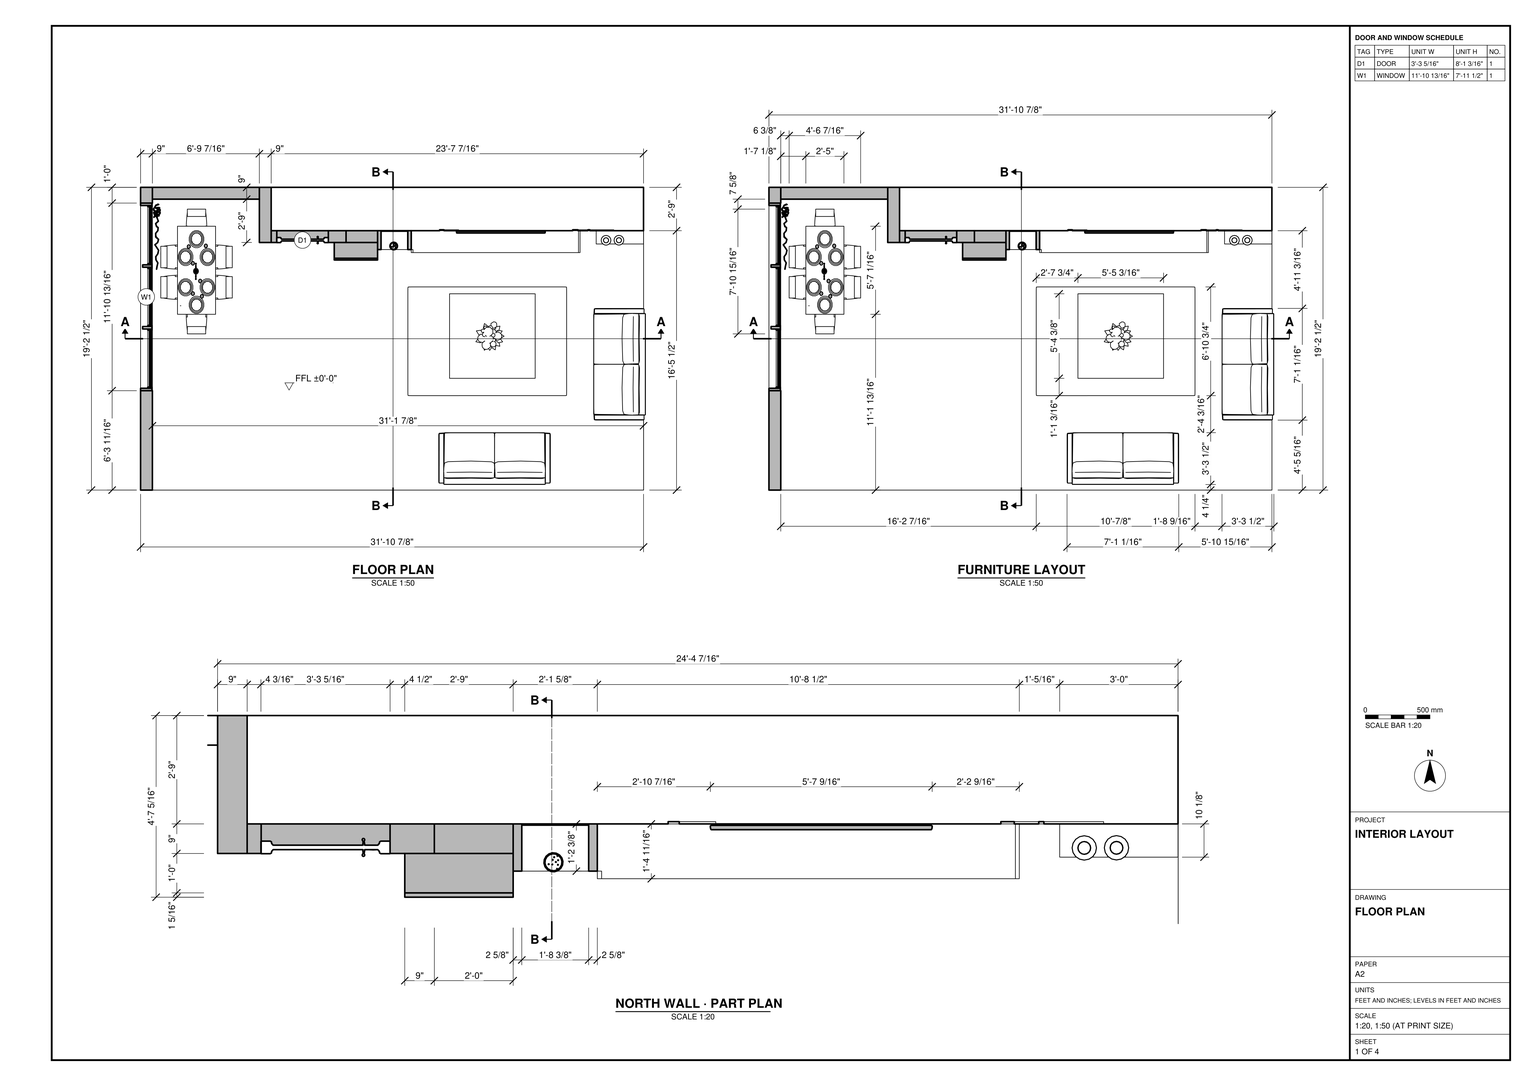
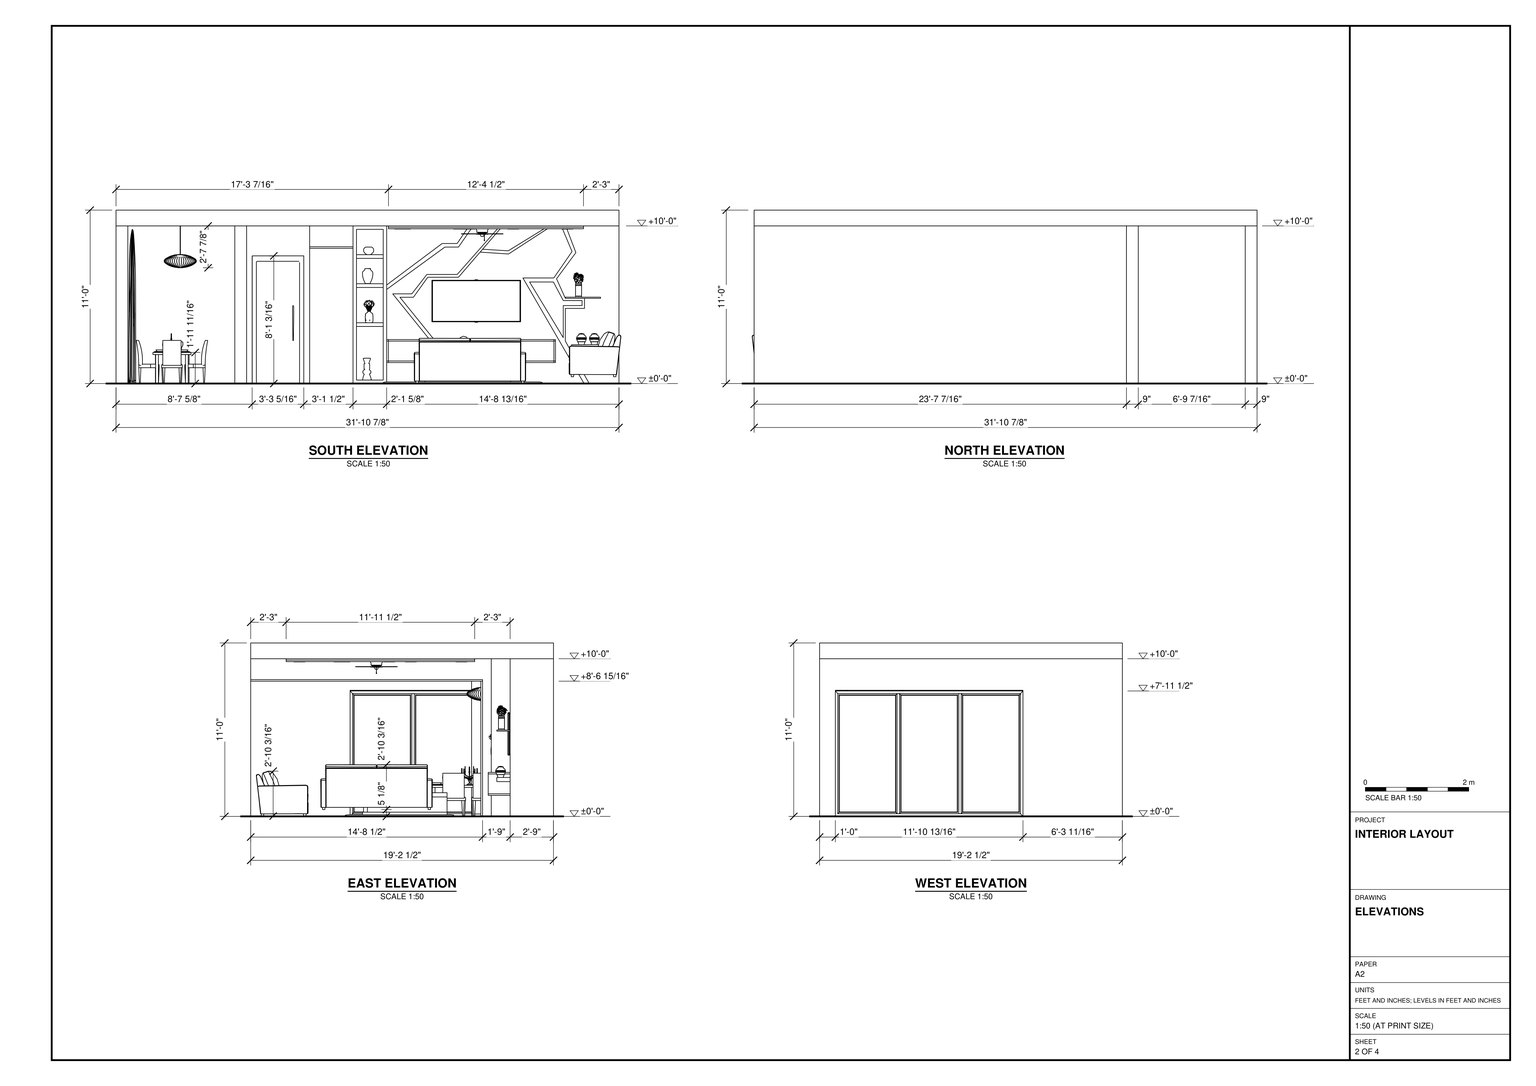
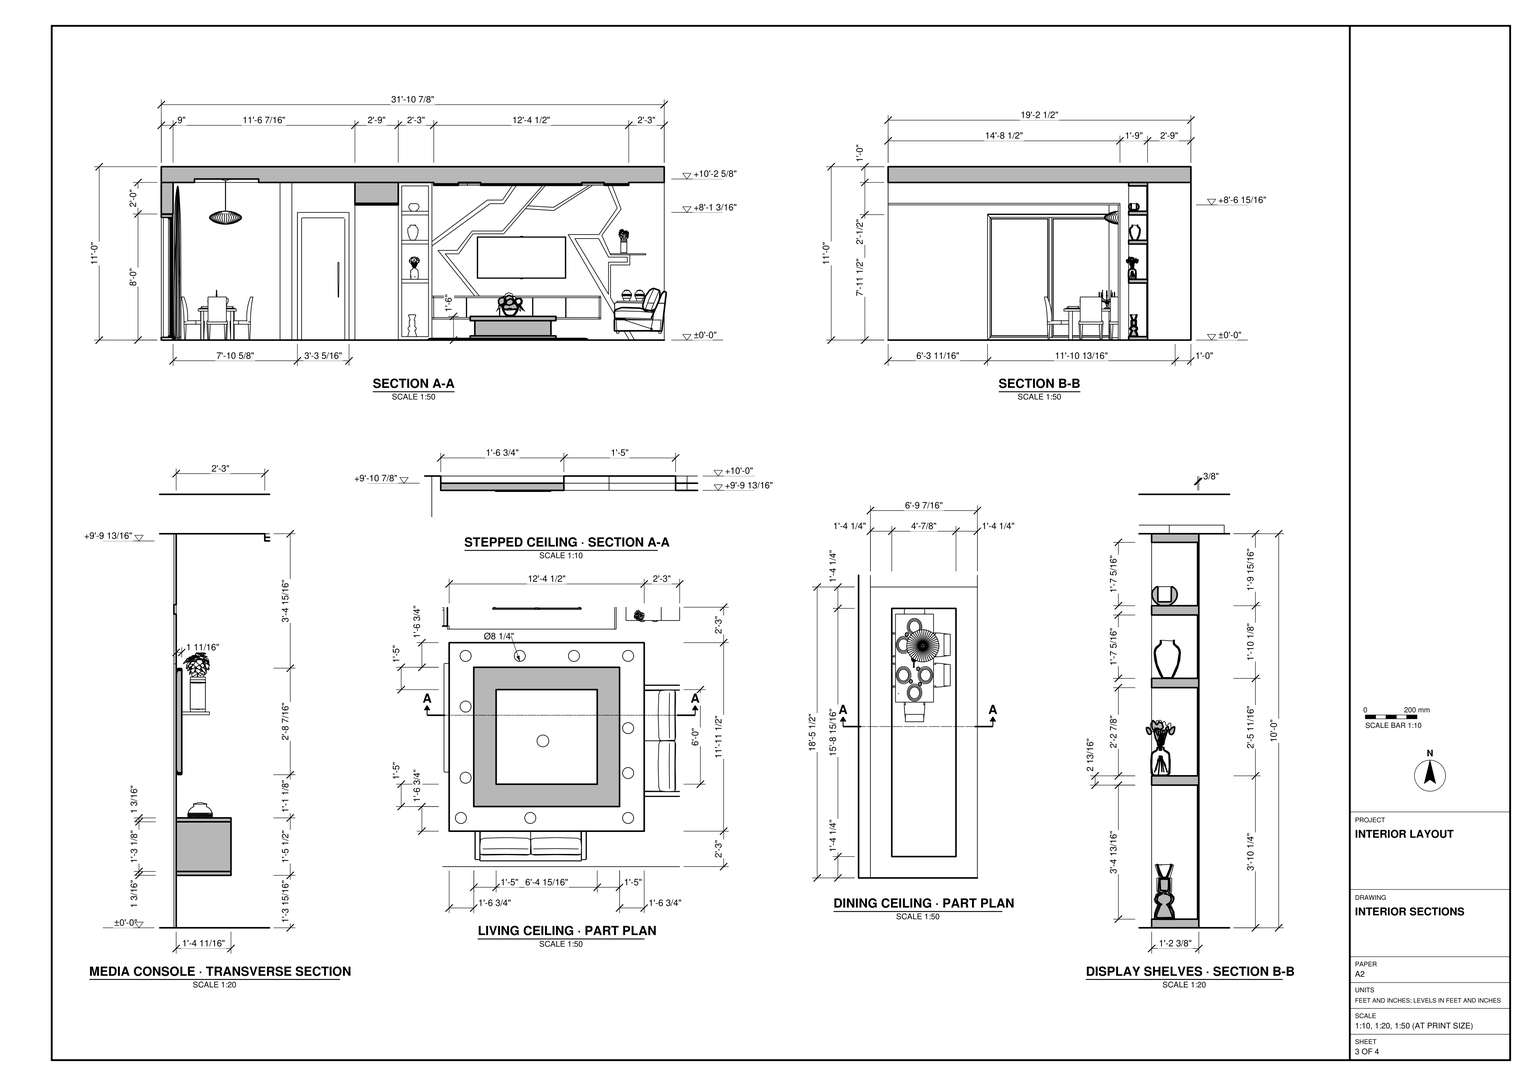
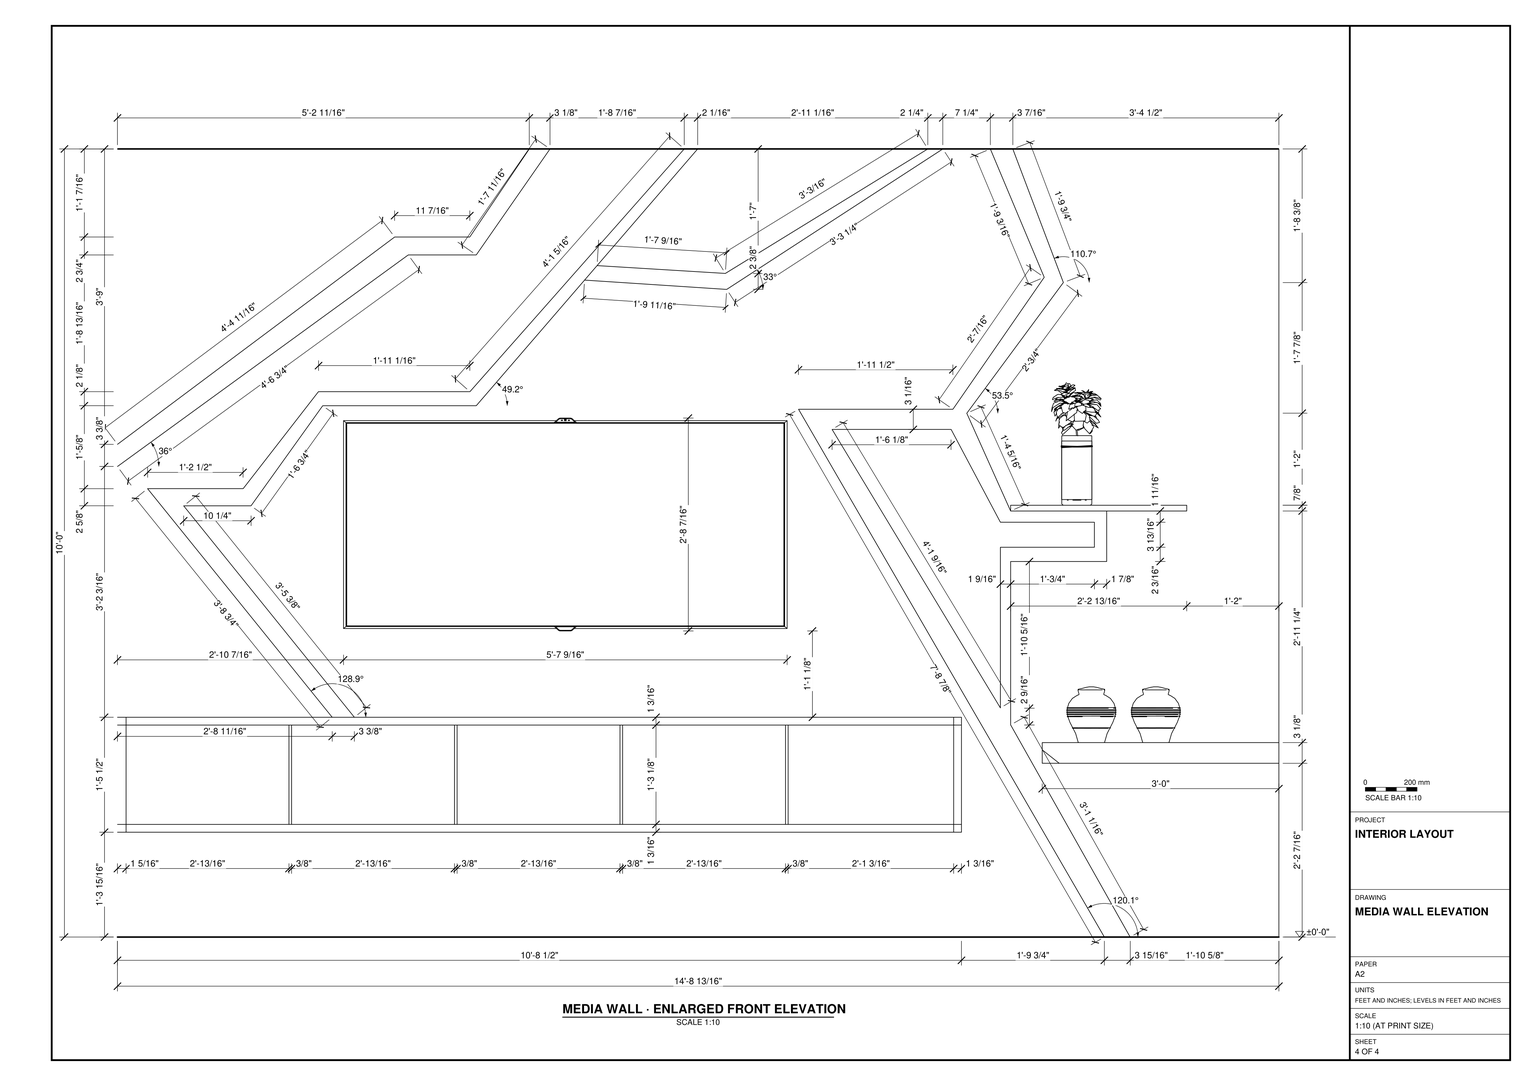
Build the furnished interior in SketchUp using task_files/diagram_01.pdf. Work in feet and inches. Set the finished floor at ±0'-0" and make the overall model 32'-3/8" along the x-axis, 19'-2 1/2" along the y-axis and 11'-0" high.

Follow the floor plan for the floor, the west window wall and the stepped north wall. Use the wall thicknesses shown, including the 9" wall returns. Fit the three-panel window beside the dining area and the single door in the north wall recess. Model the overhead slab with its main underside at +10'-0". Use the ceiling plans and sections to form the stepped rectangular ceiling over the living area and the long inset panel over the dining area.

Arrange the dining table and chairs by the window. Place the two sofas at right angles around the coffee table and rug. On the north wall, model the tall open display shelves, suspended media console, wall-mounted screen and angular wall detailing shown in elevation. Decor and loose items, including curtains, lights, the rug, tableware and shelf objects, may be any suitable library components.

Keep the walls, floor and overhead slab separate as groups or components. Make each furniture or joinery piece a separate group or component and use components for repeated parts. Save one SketchUp model as output_files/living_and_dining_interior_with_a_built_in_media_wall.skp.

# SketchUp Ruby script. Lengths in inches.
U = 1.inch
M = Sketchup.active_model
def pt(a) = Geom::Point3d.new(a.map { |v| v * U })
def face(e, loops, mat)
  f = e.add_face(loops[0].map { |a| pt(a) })
  loops[1..].each { |l| e.add_face(l.map { |a| pt(a) }).erase! }
  f.material = f.back_material = mat if mat
  f
end
# faces: each face lists its corners as indices into pts; further lists are holes
def faces(e, pts, list, mat = nil) = list.each { |f| face(e, (f[0].is_a?(Array) ? f : [f]).map { |l| l.map { |i| pts[i] } }, mat) }
# xy, xz, yz: faces in a plane at the given z, y or x. An outline is a flat list of corners, or four numbers for a rectangle; further outlines are holes
def ring(l) = l.size == 4 ? [[l[0], l[1]], [l[2], l[1]], [l[2], l[3]], [l[0], l[3]]] : l.each_slice(2).to_a
def flat(e, list, mat, &to3) = list.each { |f| face(e, (f[0].is_a?(Array) ? f : [f]).map { |l| ring(l).map { |u, v| to3.(u, v) } }, mat) }
def xy(e, z, list, mat = nil) = flat(e, list, mat) { |x, y| [x, y, z] }
def xz(e, y, list, mat = nil) = flat(e, list, mat) { |x, z| [x, y, z] }
def yz(e, x, list, mat = nil) = flat(e, list, mat) { |y, z| [x, y, z] }
def lines(e, pts, list) = list.each { |a, b| e.add_line(pt(pts[a]), pt(pts[b])) }
# prism: a flat outline (further loops are holes) pulled along v
def prism(e, loops, v, mat = nil)
  f = face(e, loops, mat); d = Geom::Vector3d.new(v.map { |x| x * U })
  f.pushpull(f.normal.samedirection?(d) ? d.length : -d.length)
end
def box(e, o, s, mat = nil) = prism(e, [[o, [o[0] + s[0], o[1], o[2]], [o[0] + s[0], o[1] + s[1], o[2]], [o[0], o[1] + s[1], o[2]]]], [0, 0, s[2]], mat)
def at(x, y, z, deg = 0) = Geom::Transformation.translation(pt([x, y, z])) * Geom::Transformation.rotation(ORIGIN, Z_AXIS, deg.degrees)
def axes(o, x, y, z) = Geom::Transformation.new([*x, 0, *y, 0, *z, 0, *pt(o).to_a, 1])
def part(name) = M.definitions.add(name)
# library, detail: a bought-in or finely detailed component or shape, given as its bounding box
def library(name, o, s) = part(name).tap { |d| box(d.entities, o, s) }
def detail(e, o, s) = box(e.add_group.entities, o, s)
def put(e, d, t, mat = nil) = e.add_instance(d, t).tap { |i| i.material = mat if mat }
def group(e, t, mat = nil) = e.add_group.tap { |g| g.transformation = t; g.material = mat if mat }.entities
root = M.entities
M.materials.add("Emissive").color = [230, 227, 173]
M.materials.add("[Color F02]").color = [204, 255, 153]
M.materials.add("[Sandstone]").color = [118, 81, 52]
M.materials.add("[Wood Veneer 01]").color = [120, 70, 37]
c1 = library("Dining Table",[54.55,57.53,0],[71.62,106.71,46.43])
c2 = library("Curtains 003",[-24.98,-2.79,0.01],[49.96,5.58,117.31])
c3 = library("Window 46-47",[-61.02,-2.17,0],[122.04,4.34,74.02])
c4 = library("Couch Potato Lite Sofa",[-42.52,-18.39,0],[85.04,39.49,34.18])
c5 = library("Pendant 001",[-12.3,-12.27,-34.51],[24.6,24.54,34.51])
c6 = library("Tlon Light 1950 Ceiling 152 010",[-38.39,-38.39,-3.78],[76.78,76.78,3.41])
c7 = library("Potted Basil 50-07",[-3.85,-3.53,0.03],[7.56,8,18.65])
c8 = library("Fan 90-20",[-15.86,-15.86,-9.19],[31.73,31.72,9.19])
c9 = library("Vase 014",[-3.77,-3.77,0],[7.54,7.54,8.49])
c10 = library("Rug 293 007",[-90.2,-61.78,-0.71],[180.4,123.56,1.82])
c11 = library("Door 243 053",[-21.6,-2.79,-0.07],[43.2,5.58,82.64])
c12 = library("Vase 296 007 003",[-3.87,-3.86,-0.02],[7.74,7.71,5.84])
c13 = library("Vase 293 004 008",[-3.27,-3.11,-0.05],[6.67,6.28,16.74])
c14 = library("Vase Tulips 12",[-3.9,-4.34,0],[7.8,8.68,17.22])
c15 = library("Vase 017",[-3.98,-3.95,0],[7.96,7.89,11.62])
c16 = library("Flat screen television",[0,1.41,1.14],[35.92,0.28,20.21])
c17 = library("Vase 008",[-10.64,-10.96,0.22],[21.74,21.78,17.78])
xy(root,0,[[0,0,9,75.6875],[9,0,382.92,0,382.92,197.5,360.23,197.5,360.23,198.1875,356.3,198.1875,356.3,197.5,206.05,197.5,206.05,183.125,180.42,183.125,180.42,175.1875,147.42,175.1875,147.42,188.5,142.94,188.5,142.94,197.5,103.69,197.5,103.69,188.5,90.42,188.5,90.42,221.5,9,221.5],[147.42,175.1875,156.42,176.5],[156.42,175.1875,180.42,176.5],[147.42,176.5,156.42,188.5],
  [156.42,176.5,180.42,188.5],[180.42,183.125,206.05,197.5],[90.42,188.5,99.42,230.5],[99.42,188.5,103.69,197.5],[142.94,188.5,156.42,197.5],
  [156.42,188.5,180.42,197.5],[99.42,197.5,356.3,197.5,356.3,198.1875,360.23,198.1875,360.23,197.5,382.875,197.5,382.875,230.5,99.42,230.5],[0,218.5,9,230.5],[9,221.5,90.42,230.5]])
xy(root,1.21,[[235.21,85.09,300.4,149.47]])
xy(root,2.63,[[183.06,183.125,203.42,197.125]],"[Wood Veneer 01]")
xy(root,3.21,[[235.21,85.09,238.71,149.47],[238.71,85.09,278.85,85.91],[278.85,85.09,278.85,88.84,297.9,88.84,297.9,87.59,300.4,87.59,300.4,85.09],[238.71,85.91,238.71,149.47,296.65,149.47,296.65,88.84,278.85,88.84,278.85,85.91],[297.9,87.59,297.9,88.84,296.65,88.84,296.65,149.47,300.4,149.47,300.4,87.59]])
xy(root,14.78,[[235.21,85.09,238.71,149.47],[238.71,85.09,278.85,85.91],[278.85,85.09,278.85,88.84,297.9,88.84,297.9,87.59,300.4,87.59,300.4,85.09],[238.71,85.91,238.71,149.47,296.65,149.47,296.65,88.84,278.85,88.84,278.85,85.91],[297.9,87.59,297.9,88.84,296.65,88.84,296.65,149.47,300.4,149.47,300.4,87.59]])
xy(root,15.96,[[206.05,180.8125,207.36,183.125],[207.36,180.8125,207.36,183.125,206.05,183.125,206.05,197.5,333.36,197.5,333.36,180.8125],[333.36,180.8125,334.55,197.5]],"[Wood Veneer 01]")
xy(root,17.15,[[206.05,180.8125,207.36,183.125],[207.36,180.8125,333.36,180.8125,333.36,197.5,206.05,197.5,206.05,183.125,207.36,183.125],[333.36,180.8125,334.55,197.5]])
xy(root,18.03,[[235.21,85.09,300.4,149.47]])
xy(root,26.46,[[346.85,187.375,349.4375,197.5],[349.4375,187.375,382.875,197.5]])
xy(root,29.61,[[346.85,187.375,382.875,197.5]])
xy(root,32.28,[[206.05,180.8125,207.36,183.125],[207.36,180.8125,207.36,183.125,206.05,183.125,206.05,197.5,333.36,197.5,333.36,180.8125],[333.36,180.8125,334.55,197.5]])
xy(root,33.46,[[238.74,197.5,242.12,198.1875]])
xy(root,33.46,[[206.05,180.8125,207.36,183.125],[207.36,180.8125,333.36,180.8125,333.36,197.5,206.05,197.5,206.05,183.125,207.36,183.125],[333.36,180.8125,334.55,197.5]],"[Wood Veneer 01]")
xy(root,43.44,[[183.06,195.125,203.42,197.125]],"Emissive")
xy(root,43.44,[[183.06,183.125,203.42,195.125]],"[Sandstone]")
xy(root,46.27,[[183.06,183.125,203.42,197.125]],"[Wood Veneer 01]")
xy(root,57.18,[[342.03,197.5,356.66,198.1875]],"Emissive")
xy(root,59.35,[[340.48,197.5,354.79,198.1875]],"Emissive")
xy(root,63.16,[[340.48,197.5,354.79,198.1875]],"Emissive")
xy(root,64.87,[[342.03,187.375,356.66,198.1875],[356.66,187.375,368.85,197.5]],"[Wood Veneer 01]")
xy(root,65.66,[[216.13,197.5,226.38,198.1875]],"Emissive")
xy(root,65.74,[[342.03,187.375,368.85,197.5]],"[Wood Veneer 01]")
xy(root,68.28,[[210.625,197.5,225.1875,198.1875]],"Emissive")
xy(root,73.13,[[183.06,195.125,203.42,197.125]],"Emissive")
xy(root,73.13,[[183.06,183.125,203.42,195.125]],"[Wood Veneer 01]")
xy(root,75.96,[[183.06,183.125,203.42,197.125]],"[Wood Veneer 01]")
xy(root,77.29,[[314.85,197.5,332.97,198.1875]],"Emissive")
xy(root,80.36,[[309.74,197.5,333.24,198.1875]],"Emissive")
xy(root,80.9,[[237.3,197.5,260.67,198.1875]],"Emissive")
xy(root,83.04,[[236.65,197.5,259.71,198.1875]],"Emissive")
xy(root,95.25,[[183.06,195.125,203.42,197.125]],"Emissive")
xy(root,95.25,[[183.06,183.125,203.42,195.125]],"[Wood Veneer 01]")
xy(root,96,[[0,75.6875,9,218.5]])
xy(root,97.1875,[[103.69,188.5,142.94,197.5]])
xy(root,98.08,[[183.06,183.125,203.42,197.125]],"[Wood Veneer 01]")
xy(root,102.92,[[147.42,175.1875,180.42,176.5]])
xy(root,102.92,[[147.42,0,180.42,175.1875]],"[Wood Veneer 01]")
xy(root,103.86,[[250.32,197.5,260.67,198.1875]],"Emissive")
xy(root,104.11,[[147.42,0,180.42,176.5]])
xy(root,106.59,[[248.25,197.5,259.69,198.1875]],"Emissive")
xy(root,117.37,[[183.06,195.125,203.42,197.125]],"Emissive")
xy(root,117.37,[[183.06,183.125,203.42,195.125]],"[Wood Veneer 01]")
xy(root,117.8125,[[[207.41,26.99,355.89,170.51],[226.16,45.74,337.14,151.76]],[243.17,62.74,320.13,134.76]])
xy(root,118.91,[[[207.41,26.99,355.89,170.51],[226.16,45.74,337.14,151.76]],[243.17,62.74,320.13,134.76]])
xy(root,120,[[0,0,9,230.5],[[9,0,90.42,221.5],[25.28,16.28,74.14,205.22]],[90.42,0,99.42,188.5],[99.42,0,147.42,188.5],[147.42,0,156.42,188.5],
  [156.42,0,180.42,188.5],[[180.42,0,180.42,183.125,206.05,183.125,206.05,197.5,268.75,197.5,268.75,198.1875,271.9,198.1875,271.9,197.5,292.34,197.5,292.34,198.1875,294.39,198.1875,294.39,197.5,329.43,197.5,329.43,198.1875,331.71,198.1875,331.71,197.5,338.94,197.5,338.94,198.1875,342.36,198.1875,342.36,197.5,382.875,197.5,382.875,0],[207.41,26.99,355.89,170.51]],[[226.16,45.74,337.14,151.76],[243.17,62.74,320.13,134.76]],[180.42,183.125,206.05,197.5],[90.42,188.5,99.42,230.5],
  [99.42,188.5,156.42,197.5],[156.42,188.5,180.42,197.5],[156.42,188.5,180.42,197.5],[99.42,197.5,99.42,230.5,382.875,230.5,382.875,197.5,342.36,197.5,342.36,198.1875,338.94,198.1875,338.94,197.5,331.71,197.5,331.71,198.1875,329.43,198.1875,329.43,197.5,294.39,197.5,294.39,198.1875,292.34,198.1875,292.34,197.5,271.9,197.5,271.9,198.1875,268.75,198.1875,268.75,197.5],[9,221.5,90.42,230.5]])
xy(root,122.625,[[25.28,16.28,74.14,205.22]])
xy(root,132,[[0,0,382.875,230.5]])
xz(root,0,[[0,0,9,120],[147.42,102.92,180.42,104.11],[147.42,104.11,180.42,120],[0,120,382.875,132]])
xz(root,16.28,[[25.28,120,74.14,122.625]])
xz(root,26.99,[[207.41,117.8125,355.89,118.91]])
xz(root,26.99,[[207.41,118.91,355.89,120]],"Emissive")
xz(root,45.74,[[226.16,117.8125,337.14,118.91],[226.16,118.91,337.14,120]])
xz(root,62.74,[[243.17,117.8125,320.13,118.91]])
xz(root,62.74,[[243.17,118.91,320.13,120]],"Emissive")
xz(root,75.6875,[[0,0,9,96]])
xz(root,85.09,[[235.21,1.21,300.4,3.21],[235.21,14.78,300.4,18.03]])
xz(root,85.91,[[238.71,3.21,278.85,14.78]])
xz(root,88.84,[[278.85,3.21,296.65,14.78]])
xz(root,134.76,[[243.17,117.8125,244.91,118.91],[244.91,117.8125,267.4,118.91],[267.4,117.8125,304.73,118.91],[304.73,117.8125,315.37,118.91],[315.37,117.8125,320.13,118.91]])
xz(root,134.76,[[243.17,118.91,244.91,120],[244.91,118.91,267.4,120],[267.4,118.91,304.73,120],[304.73,118.91,315.37,120],[315.37,118.91,320.13,120]],"Emissive")
xz(root,149.47,[[235.21,1.21,300.4,3.21],[238.71,3.21,296.65,14.78],[235.21,14.78,300.4,18.03]])
xz(root,151.76,[[226.16,117.8125,233.04,118.91],[233.04,117.8125,244.91,118.91],[244.91,117.8125,267.4,118.91],[267.4,117.8125,304.73,118.91],[304.73,117.8125,315.37,118.91],
  [315.37,117.8125,337.14,118.91]])
xz(root,151.76,[[226.16,118.91,233.04,120],[233.04,118.91,244.91,120],[244.91,118.91,267.4,120],[267.4,118.91,304.73,120],[304.73,118.91,315.37,120],
  [315.37,118.91,337.14,120]],"Emissive")
xz(root,170.51,[[207.41,117.8125,233.04,118.91],[233.04,117.8125,244.91,118.91],[244.91,117.8125,267.4,118.91],[267.4,117.8125,304.73,118.91],[304.73,117.8125,315.37,118.91],
  [315.37,117.8125,355.89,118.91]])
xz(root,170.51,[[207.41,118.91,233.04,120],[233.04,118.91,244.91,120],[244.91,118.91,267.4,120],[267.4,118.91,304.73,120],[304.73,118.91,315.37,120],
  [315.37,118.91,355.89,120]],"Emissive")
xz(root,175.1875,[[147.42,0,180.42,102.92]],"[Wood Veneer 01]")
xz(root,176.5,[[147.42,0,180.42,102.92],[147.42,102.92,180.42,104.11]])
xz(root,180.8125,[[207.36,17.15,232.16,32.28],[232.16,17.15,232.5625,32.28],[232.5625,17.15,257.36,32.28],[257.36,17.15,257.76,32.28],[257.76,17.15,282.5625,32.28],
  [282.5625,17.15,282.96,32.28],[282.96,17.15,307.76,32.28],[307.76,17.15,308.16,32.28],[308.16,17.15,333.36,32.28]])
xz(root,180.8125,[[206.05,15.96,207.36,17.15],[207.36,15.96,333.36,17.15],[333.36,15.96,334.55,17.15],[206.05,17.15,207.36,32.28],[333.36,17.15,334.55,32.28],
  [206.05,32.28,207.36,33.46],[207.36,32.28,333.36,33.46],[333.36,32.28,334.55,33.46]],"[Wood Veneer 01]")
xz(root,183.125,[[206.05,15.96,207.36,17.15],[206.05,17.15,207.36,32.28],[206.05,32.28,207.36,33.46]])
xz(root,183.125,[[[180.42,0,206.05,120],[183.06,2.63,203.42,117.37]],[183.06,43.44,203.42,46.27],[183.06,73.13,203.42,75.96],[183.06,95.25,203.42,98.08]],"[Wood Veneer 01]")
xz(root,187.375,[[346.85,26.46,349.4375,26.46,346.85,28.5],[349.4375,26.46,382.875,26.46,382.875,29.61,346.85,29.61,346.85,28.5]])
xz(root,187.375,[[342.03,64.87,368.85,65.74]],"[Wood Veneer 01]")
xz(root,188.5,[[90.42,0,99.42,120],[99.42,0,103.69,0,103.69,97.1875,142.94,97.1875,142.94,0,147.42,0,147.42,120,99.42,120],[147.42,0,156.42,120],[156.42,0,180.42,120]])
xz(root,197.125,[[183.06,2.63,203.42,43.44],[183.06,46.27,203.42,73.13],[183.06,75.96,203.42,95.25],[183.06,98.08,203.42,117.37]],"[Wood Veneer 01]")
xz(root,197.5,[[99.42,0,103.69,120],[103.69,0,142.94,97.1875],[142.94,0,156.42,120],[156.42,0,180.42,120],[180.42,0,206.05,120],
  [206.05,0,356.3,0,309.74,80.36,333.24,80.36,347.15,100.46,338.94,120,331.71,120,298.81,98.61,277.17,100.03,260.67,80.9,237.3,80.9,226.38,65.66,216.13,65.66,242.12,33.46,334.55,33.46,334.55,15.96,206.05,15.96],[382.875,0,382.92,0,382.875,0.04],[206.05,15.96,333.36,17.15],[333.36,15.96,334.55,17.15],[206.05,17.15,333.36,32.28],
  [333.36,17.15,334.55,32.28],[346.85,26.46,346.85,28.5,349.4375,26.46],[349.4375,26.46,346.85,28.5,346.85,29.61,382.875,29.61,382.875,26.46],[206.05,32.28,333.36,33.46],[333.36,32.28,334.55,33.46],
  [340.48,34.89,340.48,59.35,354.79,59.35,354.79,63.16,340.48,63.16,332.97,77.29,314.85,77.29],[206.05,75.02,248.25,106.59,259.69,106.59,268.75,120,206.05,120],[103.69,97.1875,142.94,120]])
xz(root,197.5,[[206.05,33.46,238.74,33.46,210.625,68.28,225.1875,68.28,236.65,83.04,259.71,83.04,292.34,120,271.9,120,260.67,103.86,250.32,103.86,206.05,71.65]],"[Color F02]")
xz(root,197.5,[[[360.23,0,382.875,0,382.875,0.04,382.92,0,382.875,0,382.875,26.46,346.85,26.46,346.85,29.61,382.875,29.61,382.875,120,342.36,120,350.0625,99.66,335.36,79.75,342.03,64.87,342.03,65.74,368.85,65.74,368.85,64.87,356.66,64.87,356.66,57.18,342.03,57.18,342.03,32.31],[346.85,26.46,346.85,28.5,349.4375,26.46]],[298.6,101.04,329.43,120,294.39,120,280.99,104.46,279.07,102.23]],"[Sandstone]")
xz(root,198.1875,[[[356.3,0,360.23,0,342.03,32.31,342.03,57.18,356.66,57.18,356.66,64.87,342.03,64.87,335.36,79.75,350.0625,99.66,342.36,120,338.94,120,347.15,100.46,333.24,80.36,309.74,80.36],[340.48,34.89,314.85,77.29,332.97,77.29,340.48,63.16,354.79,63.16,354.79,59.35,340.48,59.35]],[238.74,33.46,242.12,33.46,216.13,65.66,226.38,65.66,237.3,80.9,260.67,80.9,277.17,100.03,279.07,102.23,280.99,104.46,294.39,120,292.34,120,259.71,83.04,236.65,83.04,225.1875,68.28,210.625,68.28],[206.05,71.65,250.32,103.86,260.67,103.86,271.9,120,268.75,120,259.69,106.59,248.25,106.59,206.05,75.02],[298.81,98.61,331.71,120,329.43,120,298.6,101.04,279.07,102.23,277.17,100.03]])
xz(root,205.22,[[25.28,120,74.14,122.625]])
xz(root,218.5,[[0,0,9,96]])
xz(root,221.5,[[9,0,90.42,120]])
xz(root,230.5,[[0,0,9,120],[9,0,90.42,120],[90.42,0,99.42,120],[99.42,0,382.875,120],[0,120,382.875,132]])
yz(root,0,[[0,0,0,120,230.5,120,230.5,0,218.5,0,218.5,96,75.6875,96,75.6875,0],[0,120,230.5,132]])
yz(root,9,[[0,0,75.6875,0,75.6875,96,218.5,96,218.5,0,221.5,0,221.5,120,0,120],[221.5,0,230.5,120]])
yz(root,25.28,[[16.28,120,205.22,122.625]])
yz(root,74.14,[[16.28,120,188.5,122.625],[188.5,120,205.22,122.625]])
yz(root,90.42,[[188.5,0,221.5,120],[221.5,0,230.5,120]])
yz(root,99.42,[[188.5,0,197.5,120],[197.5,0,230.5,120]])
yz(root,103.69,[[188.5,0,197.5,97.1875]])
yz(root,142.94,[[188.5,0,197.5,97.1875]])
yz(root,147.42,[[176.5,0,176.5,104.11,0,104.11,0,120,188.5,120,188.5,0]])
yz(root,147.42,[[175.1875,0,176.5,102.92],[0,102.92,176.5,104.11]],"[Wood Veneer 01]")
yz(root,156.42,[[188.5,0,197.5,120]])
yz(root,180.42,[[176.5,0,183.125,0,183.125,120,0,120,0,104.11,176.5,104.11],[183.125,0,188.5,120],[188.5,0,197.5,120]])
yz(root,180.42,[[175.1875,0,176.5,102.92],[0,102.92,176.5,104.11]],"[Wood Veneer 01]")
yz(root,183.06,[[183.125,2.63,197.125,43.44],[183.125,46.27,197.125,73.13],[183.125,75.96,197.125,95.25],[183.125,98.08,197.125,117.37]],"[Wood Veneer 01]")
yz(root,203.42,[[183.125,2.63,197.125,15.96],[183.125,15.96,197.125,17.15],[183.125,17.15,197.125,32.28],[183.125,32.28,197.125,33.46],[183.125,33.46,197.125,43.44],
  [183.125,46.27,197.125,73.13],[183.125,75.96,197.125,95.25],[183.125,98.08,197.125,117.37]],"[Wood Veneer 01]")
yz(root,206.05,[[183.125,0,197.5,15.96],[183.125,15.96,197.5,17.15],[183.125,17.15,197.5,32.28],[183.125,32.28,197.5,33.46]])
yz(root,206.05,[[197.5,71.65,198.1875,75.02]],"Emissive")
yz(root,206.05,[[180.8125,15.96,183.125,17.15],[180.8125,17.15,183.125,32.28],[180.8125,32.28,183.125,33.46],[183.125,33.46,197.5,120]],"[Wood Veneer 01]")
yz(root,207.36,[[180.8125,15.96,183.125,17.15],[180.8125,17.15,183.125,32.28],[180.8125,32.28,183.125,33.46]])
yz(root,207.41,[[26.99,117.8125,170.51,118.91]])
yz(root,207.41,[[26.99,118.91,170.51,120]],"Emissive")
yz(root,226.16,[[45.74,117.8125,151.76,118.91]])
yz(root,226.16,[[45.74,118.91,151.76,120]],"Emissive")
yz(root,235.21,[[85.09,1.21,149.47,3.21],[85.09,14.78,149.47,18.03]])
yz(root,238.71,[[85.91,3.21,149.47,14.78]])
yz(root,243.17,[[62.74,117.8125,134.76,118.91]])
yz(root,243.17,[[62.74,118.91,134.76,120]],"Emissive")
yz(root,278.85,[[85.91,3.21,88.84,14.78]])
yz(root,296.65,[[88.84,3.21,149.47,14.78]])
yz(root,300.4,[[85.09,1.21,149.47,3.21],[85.09,14.78,149.47,18.03]])
yz(root,320.13,[[62.74,117.8125,134.76,118.91]])
yz(root,320.13,[[62.74,118.91,134.76,120]],"Emissive")
yz(root,333.36,[[180.8125,15.96,197.5,17.15],[180.8125,17.15,197.5,32.28],[180.8125,32.28,197.5,33.46]])
yz(root,334.55,[[180.8125,32.28,197.5,33.46]],"[Sandstone]")
yz(root,334.55,[[180.8125,15.96,197.5,17.15],[180.8125,17.15,197.5,32.28]],"[Wood Veneer 01]")
yz(root,337.14,[[45.74,117.8125,151.76,118.91]])
yz(root,337.14,[[45.74,118.91,151.76,120]],"Emissive")
yz(root,340.48,[[197.5,34.89,198.1875,59.35]],"Emissive")
yz(root,342.03,[[197.5,32.31,198.1875,57.18]],"Emissive")
yz(root,342.03,[[187.375,64.87,197.5,65.74]],"[Wood Veneer 01]")
yz(root,346.85,[[187.375,26.46,197.5,28.5],[187.375,28.5,197.5,29.61]])
yz(root,354.79,[[197.5,59.35,198.1875,63.16]],"Emissive")
yz(root,355.89,[[26.99,117.8125,170.51,118.91]])
yz(root,355.89,[[26.99,118.91,170.51,120]],"Emissive")
yz(root,356.66,[[197.5,57.18,198.1875,64.87]],"Emissive")
yz(root,368.85,[[187.375,64.87,197.5,65.74]],"[Wood Veneer 01]")
yz(root,382.875,[[197.5,0,230.5,120],[187.375,26.46,197.5,29.61],[0,120,230.5,132]])
p = [[309.74,197.5,80.36],[356.3,197.5,0],[356.3,198.1875,0],[309.74,198.1875,80.36],[360.23,197.5,0],[342.03,197.5,32.31],
  [342.03,198.1875,32.31],[360.23,198.1875,0],[346.85,197.5,28.5],[349.4375,197.5,26.46],[349.4375,187.375,26.46],[346.85,187.375,28.5],
  [210.625,197.5,68.28],[238.74,197.5,33.46],[238.74,198.1875,33.46],[210.625,198.1875,68.28],[242.12,197.5,33.46],[216.13,197.5,65.66],
  [216.13,198.1875,65.66],[242.12,198.1875,33.46],[340.48,197.5,34.89],[314.85,197.5,77.29],[314.85,198.1875,77.29],[340.48,198.1875,34.89],
  [332.97,197.5,77.29],[340.48,197.5,63.16],[340.48,198.1875,63.16],[332.97,198.1875,77.29],[342.03,197.5,64.87],[335.36,197.5,79.75],
  [335.36,198.1875,79.75],[342.03,198.1875,64.87],[226.38,197.5,65.66],[237.3,197.5,80.9],[237.3,198.1875,80.9],[226.38,198.1875,65.66],
  [236.65,197.5,83.04],[225.1875,197.5,68.28],[225.1875,198.1875,68.28],[236.65,198.1875,83.04],[206.05,197.5,71.65],[250.32,197.5,103.86],
  [250.32,198.1875,103.86],[206.05,198.1875,71.65],[248.25,197.5,106.59],[206.05,197.5,75.02],[206.05,198.1875,75.02],[248.25,198.1875,106.59],
  [350.0625,197.5,99.66],[350.0625,198.1875,99.66],[347.15,197.5,100.46],[333.24,197.5,80.36],[333.24,198.1875,80.36],[347.15,198.1875,100.46],
  [277.17,197.5,100.03],[277.17,198.1875,100.03],[260.67,198.1875,80.9],[260.67,197.5,80.9],[292.34,197.5,120],[259.71,197.5,83.04],
  [259.71,198.1875,83.04],[292.34,198.1875,120],[298.81,197.5,98.61],[298.81,198.1875,98.61],[331.71,197.5,120],[331.71,198.1875,120],
  [342.36,197.5,120],[342.36,198.1875,120],[338.94,197.5,120],[338.94,198.1875,120],[298.6,197.5,101.04],[279.07,197.5,102.23],
  [279.07,198.1875,102.23],[298.6,198.1875,101.04],[329.43,197.5,120],[329.43,198.1875,120],[280.99,197.5,104.46],[280.99,198.1875,104.46],
  [260.67,197.5,103.86],[271.9,197.5,120],[271.9,198.1875,120],[260.67,198.1875,103.86],[294.39,197.5,120],[294.39,198.1875,120],
  [268.75,197.5,120],[259.69,197.5,106.59],[259.69,198.1875,106.59],[268.75,198.1875,120]]
faces(root,p,[[0,1,2,3],[4,5,6,7],[12,13,14,15],[16,17,18,19],[20,21,22,23],[24,25,26,27],[28,29,30,31],[32,33,34,35],
  [36,37,38,39],[40,41,42,43],[44,45,46,47],[29,48,49,30],[50,51,52,53],[54,55,56,57],[58,59,60,61],[54,62,63,55],
  [62,64,65,63],[48,66,67,49],[68,50,53,69],[70,71,72,73],[74,70,73,75],[71,76,77,72],[78,79,80,81],[76,82,83,77],
  [84,85,86,87]],"Emissive")
faces(root,p,[[8,9,10,11]])
put(root,c1,axes([-26.09,67.73,0],[0.76,0,0],[0,0.89,0],[0,0,0.82]))
put(root,c2,at(12.26,193.09,0,-90))
put(root,c3,axes([4.33,147.09,0],[0,-1.17014,0],[2,0,0],[0,0,1.29]))
put(root,c4,at(269.45,25.34,0.25,180))
put(root,c5,at(48.91,176.74,122.625))
put(root,c6,axes([216.35,37.06,118.04],[0.11,0,0],[0,0.11,0],[0,0,0.11]))
put(root,c7,at(352.11,190.9,65.72))
put(root,c8,at(278.78,95.71,117.8125))
put(root,c9,at(354.33,190.19,29.61))
put(root,c9,at(364.14,190.23,29.61))
put(root,c10,axes([263.9,113.3,0.48],[0.67,0,0],[0,0.67,0],[0,0,0.67]))
put(root,c11,axes([123.28,190.35,0.08],[0.91003,0,0],[0,1,0],[0,0,1.17617]))
put(root,c12,at(192.3125,187.07,98.08))
put(root,c13,at(190.96,187,2.63))
put(root,c14,at(192.625,185.82,46.27))
put(root,c15,at(191.56,187.88,75.96))
put(root,c4,at(363.28,95.8,5.15,-90))
put(root,c16,axes([240.47,186.66,44.77],[1.88009,0,0],[0,6.43,0],[0,0,1.60448]))
put(root,c17,at(265.625,117.33,18.03))
put(root,c6,axes([269.16,37.06,118.04],[0.11,0,0],[0,0.11,0],[0,0,0.11]))
put(root,c6,axes([343.64,37.06,118.04],[0.11,0,0],[0,0.11,0],[0,0,0.11]))
put(root,c6,axes([343.64,71.25,118.04],[0.11,0,0],[0,0.11,0],[0,0,0.11]))
put(root,c6,axes([343.64,105.43,118.04],[0.11,0,0],[0,0.11,0],[0,0,0.11]))
put(root,c6,axes([343.64,160.43,118.04],[0.11,0,0],[0,0.11,0],[0,0,0.11]))
put(root,c6,axes([302.41,160.43,118.04],[0.11,0,0],[0,0.11,0],[0,0,0.11]))
put(root,c6,axes([261.18,160.43,118.04],[0.11,0,0],[0,0.11,0],[0,0,0.11]))
put(root,c6,axes([219.95,160.43,118.04],[0.11,0,0],[0,0.11,0],[0,0,0.11]))
put(root,c6,axes([219.95,121.87,118.04],[0.11,0,0],[0,0.11,0],[0,0,0.11]))
put(root,c6,axes([219.95,67.68,118.04],[0.11,0,0],[0,0.11,0],[0,0,0.11]))
